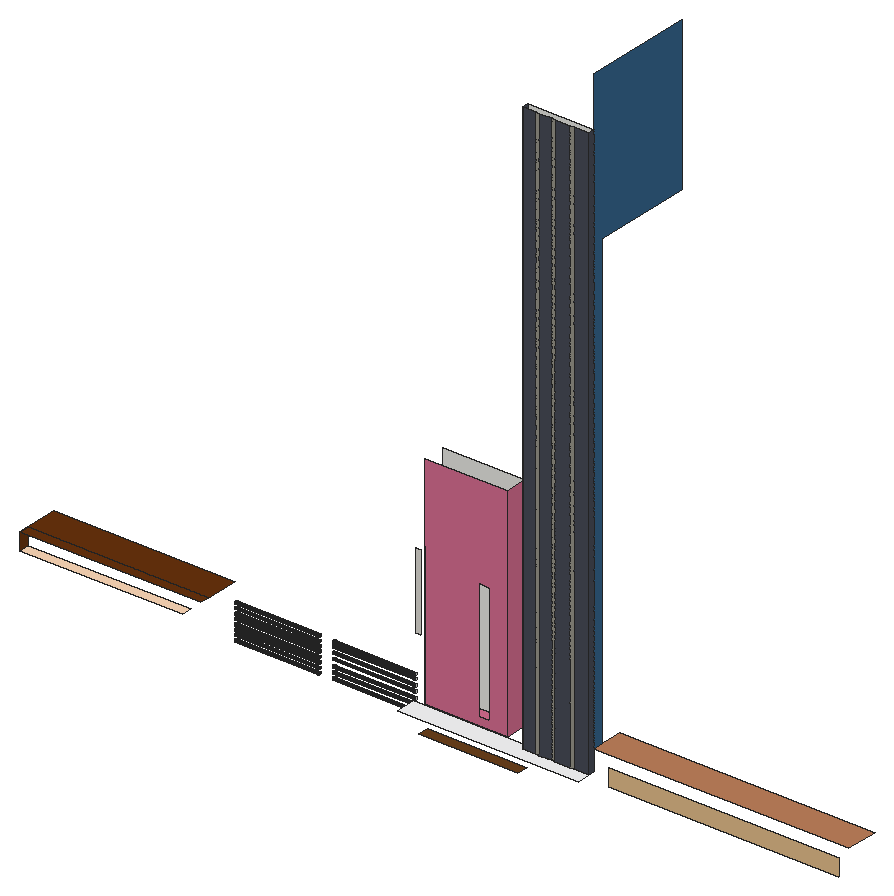
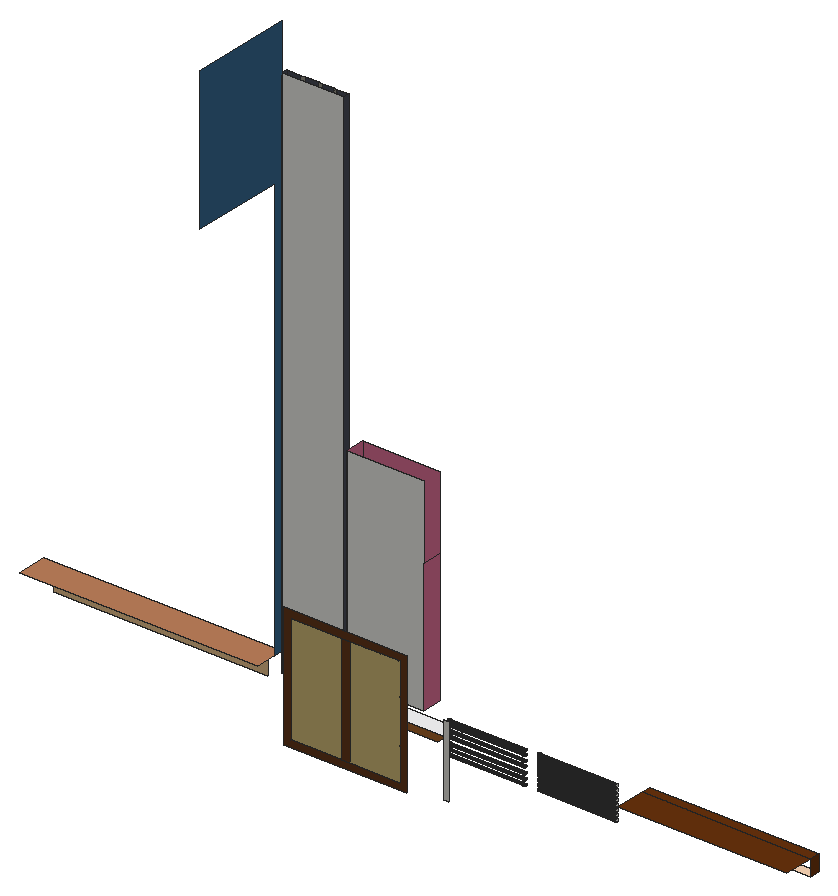
# SketchUp Ruby script. Lengths in inches.
U = 1.inch
M = Sketchup.active_model
def pt(a) = Geom::Point3d.new(a.map { |v| v * U })
def face(e, loops, mat)
  f = e.add_face(loops[0].map { |a| pt(a) })
  loops[1..].each { |l| e.add_face(l.map { |a| pt(a) }).erase! }
  f.material = f.back_material = mat if mat
  f
end
# faces: each face lists its corners as indices into pts; further lists are holes
def faces(e, pts, list, mat = nil) = list.each { |f| face(e, (f[0].is_a?(Array) ? f : [f]).map { |l| l.map { |i| pts[i] } }, mat) }
# xy, xz, yz: faces in a plane at the given z, y or x. An outline is a flat list of corners, or four numbers for a rectangle; further outlines are holes
def ring(l) = l.size == 4 ? [[l[0], l[1]], [l[2], l[1]], [l[2], l[3]], [l[0], l[3]]] : l.each_slice(2).to_a
def flat(e, list, mat, &to3) = list.each { |f| face(e, (f[0].is_a?(Array) ? f : [f]).map { |l| ring(l).map { |u, v| to3.(u, v) } }, mat) }
def xy(e, z, list, mat = nil) = flat(e, list, mat) { |x, y| [x, y, z] }
def xz(e, y, list, mat = nil) = flat(e, list, mat) { |x, z| [x, y, z] }
def yz(e, x, list, mat = nil) = flat(e, list, mat) { |y, z| [x, y, z] }
def lines(e, pts, list) = list.each { |a, b| e.add_line(pt(pts[a]), pt(pts[b])) }
# prism: a flat outline (further loops are holes) pulled along v
def prism(e, loops, v, mat = nil)
  f = face(e, loops, mat); d = Geom::Vector3d.new(v.map { |x| x * U })
  f.pushpull(f.normal.samedirection?(d) ? d.length : -d.length)
end
def box(e, o, s, mat = nil) = prism(e, [[o, [o[0] + s[0], o[1], o[2]], [o[0] + s[0], o[1] + s[1], o[2]], [o[0], o[1] + s[1], o[2]]]], [0, 0, s[2]], mat)
def at(x, y, z, deg = 0) = Geom::Transformation.translation(pt([x, y, z])) * Geom::Transformation.rotation(ORIGIN, Z_AXIS, deg.degrees)
def axes(o, x, y, z) = Geom::Transformation.new([*x, 0, *y, 0, *z, 0, *pt(o).to_a, 1])
def part(name) = M.definitions.add(name)
# library, detail: a bought-in or finely detailed component or shape, given as its bounding box
def library(name, o, s) = part(name).tap { |d| box(d.entities, o, s) }
def detail(e, o, s) = box(e.add_group.entities, o, s)
def put(e, d, t, mat = nil) = e.add_instance(d, t).tap { |i| i.material = mat if mat }
def group(e, t, mat = nil) = e.add_group.tap { |g| g.transformation = t; g.material = mat if mat }.entities
root = M.entities
M.materials.add("[0001_PaleVioletRed]").color = [211, 108, 142]
M.materials.add("[0027_PeachPuff]").color = [255, 218, 185]
M.materials.add("[0036_BurlyWood]").color = [222, 184, 135]
M.materials.add("[0043_SaddleBrown]").color = [104, 51, 14]
M.materials.add("[0100_SteelBlue]").color = [53, 99, 137]
M.materials.add("[Formica Graystone]").color = [149, 146, 135]
M.materials.add("[Formica Laminate Dark]").color = [70, 74, 84]
M.materials.add("[Polished Concrete New]").color = [200, 200, 203]
M.materials.add("[Quartz Light Grey]").color = [251, 251, 252]
M.materials.add("[Terrazzo Tile Light]").color = [219, 217, 210]
M.materials.add("[Window Covering 02]").color = [199, 178, 115]
M.materials.add("[Wood Cherry Original]").color = [96, 54, 26]
M.materials.add("[Wood Floor Parquet]").color = [107, 65, 28]
M.materials.add("[Wood Veneer 02]").color = [190, 128, 91]
xy(root,37.8125,[[216.35,107.04,269.29,112.73]],"[Wood Floor Parquet]")
xy(root,44.875,[[266.37,114.04,301.48,117.35]])
xy(root,44.875,[[205.34,107.04,301.48,107.04,301.48,114.04,266.37,114.04,266.37,117.35,205.34,117.35]],"[Quartz Light Grey]")
xy(root,47.01,[[0,112.04,86.375,117.35]],"[0027_PeachPuff]")
xy(root,53.88,[[220.625,105.92,264.66,117.35]],"[0001_PaleVioletRed]")
xy(root,56.125,[[0,112.04,96.16,117.35],[0,117.35,96.16,134.6]],"[0043_SaddleBrown]")
xy(root,56.125,[[301.48,117.35,437.01,134.6]],"[Wood Veneer 02]")
xz(root,105.92,[[[220.625,53.88,264.66,171.19],[248.98,57.97,254.98,121.72]]],"[0001_PaleVioletRed]")
xz(root,114.04,[[272.89,44.875,274.86,351.35],[281.39,44.875,283.36,351.35],[291.26,44.875,293.24,351.35]],"[Formica Graystone]")
xz(root,114.04,[[266.37,44.875,272.89,351.35],[274.86,44.875,281.39,351.35],[283.36,44.875,291.26,351.35],[293.24,44.875,301.48,351.35]],"[Formica Laminate Dark]")
xz(root,117.35,[[266.37,44.875,301.48,351.35],[220.625,53.88,264.66,171.19]])
xz(root,117.35,[[309.46,40.81,431.59,49.875]],"[0036_BurlyWood]")
xz(root,162.72,[[170.43,45.29,173.12,85.79]],"[Terrazzo Tile Light]")
xz(root,162.72,[[198.18,45.28,226.54,107.29],[230.91,45.28,260.19,107.29]],"[Window Covering 02]")
xz(root,162.72,[[[194.0625,41.16,264.3125,111.41],[198.18,45.28,260.19,107.29]],[226.54,45.28,230.91,107.29]],"[Wood Cherry Original]")
yz(root,0,[[112.04,47.01,117.35,56.125]],"[0043_SaddleBrown]")
yz(root,108.27,[[120.22,38.1,120.06,38.12,119.91,38.18,119.78,38.28,119.68,38.41,119.61,38.5625,119.59,38.72,119.61,38.88,119.68,39.04,119.78,39.16,119.91,39.26,120.06,39.33,120.22,39.35,120.38,39.33,120.53,39.26,120.66,39.16,120.76,39.04,120.82,38.88,120.84,38.72,120.82,38.5625,120.76,38.41,120.66,38.28,120.53,38.18,120.38,38.12],[120.22,40.66,120.06,40.68,119.91,40.74,119.78,40.84,119.68,40.97,119.61,41.125,119.59,41.29,119.61,41.45,119.68,41.6,119.78,41.73,119.91,41.83,120.06,41.89,120.22,41.91,120.38,41.89,120.53,41.83,120.66,41.73,120.76,41.6,120.82,41.45,120.84,41.29,120.82,41.125,120.76,40.97,120.66,40.84,120.53,40.74,120.38,40.68],[120.22,43.22,120.06,43.24,119.91,43.31,119.78,43.41,119.68,43.54,119.61,43.6875,119.59,43.85,119.61,44.01,119.68,44.16,119.78,44.29,119.91,44.39,120.06,44.45,120.22,44.47,120.38,44.45,120.53,44.39,120.66,44.29,120.76,44.16,120.82,44.01,120.84,43.85,120.82,43.6875,120.76,43.54,120.66,43.41,120.53,43.31,120.38,43.24],[120.22,45.79,120.06,45.81,119.91,45.87,119.78,45.97,119.68,46.1,119.61,46.25,119.59,46.41,119.61,46.57,119.68,46.72,119.78,46.85,119.91,46.95,120.06,47.01,120.22,47.04,120.38,47.01,120.53,46.95,120.66,46.85,120.76,46.72,120.82,46.57,120.84,46.41,120.82,46.25,120.76,46.1,120.66,45.97,120.53,45.87,120.38,45.81],[120.22,48.35,120.06,48.37,119.91,48.43,119.78,48.53,119.68,48.66,119.61,48.8125,119.59,48.97,119.61,49.13,119.68,49.29,119.78,49.41,119.91,49.51,120.06,49.58,120.22,49.6,120.38,49.58,120.53,49.51,120.66,49.41,120.76,49.29,120.82,49.13,120.84,48.97,120.82,48.8125,120.76,48.66,120.66,48.53,120.53,48.43,120.38,48.37],
  [120.22,50.91,120.06,50.93,119.91,50.99,119.78,51.09,119.68,51.22,119.61,51.375,119.59,51.54,119.61,51.7,119.68,51.85,119.78,51.98,119.91,52.08,120.06,52.14,120.22,52.16,120.38,52.14,120.53,52.08,120.66,51.98,120.76,51.85,120.82,51.7,120.84,51.54,120.82,51.375,120.76,51.22,120.66,51.09,120.53,50.99,120.38,50.93],[120.22,53.47,120.06,53.49,119.91,53.56,119.78,53.66,119.68,53.79,119.61,53.9375,119.59,54.1,119.61,54.26,119.68,54.41,119.78,54.54,119.91,54.64,120.06,54.7,120.22,54.72,120.38,54.7,120.53,54.64,120.66,54.54,120.76,54.41,120.82,54.26,120.84,54.1,120.82,53.9375,120.76,53.79,120.66,53.66,120.53,53.56,120.38,53.49],[120.22,56.04,120.06,56.06,119.91,56.12,119.78,56.22,119.68,56.35,119.61,56.5,119.59,56.66,119.61,56.82,119.68,56.97,119.78,57.1,119.91,57.2,120.06,57.26,120.22,57.29,120.38,57.26,120.53,57.2,120.66,57.1,120.76,56.97,120.82,56.82,120.84,56.66,120.82,56.5,120.76,56.35,120.66,56.22,120.53,56.12,120.38,56.06]])
yz(root,204.4,[[120.29,38.04,120.45,38.0625,120.6,38.125,120.73,38.22,120.83,38.35,120.89,38.5,120.91,38.66,120.89,38.83,120.83,38.98,120.73,39.11,120.6,39.21,120.45,39.27,120.29,39.29,120.13,39.27,119.98,39.21,119.85,39.11,119.75,38.98,119.6875,38.83,119.66,38.66,119.6875,38.5,119.75,38.35,119.85,38.22,119.98,38.125,120.13,38.0625],[120.29,41.04,120.45,41.0625,120.6,41.125,120.73,41.22,120.83,41.35,120.89,41.5,120.91,41.66,120.89,41.83,120.83,41.98,120.73,42.11,120.6,42.21,120.45,42.27,120.29,42.29,120.13,42.27,119.98,42.21,119.85,42.11,119.75,41.98,119.6875,41.83,119.66,41.66,119.6875,41.5,119.75,41.35,119.85,41.22,119.98,41.125,120.13,41.0625],[120.29,43.91,120.45,43.9375,120.6,44,120.73,44.1,120.83,44.23,120.89,44.38,120.91,44.54,120.89,44.7,120.83,44.85,120.73,44.98,120.6,45.08,120.45,45.14,120.29,45.16,120.13,45.14,119.98,45.08,119.85,44.98,119.75,44.85,119.6875,44.7,119.66,44.54,119.6875,44.38,119.75,44.23,119.85,44.1,119.98,44,120.13,43.9375],[120.29,47.41,120.45,47.4375,120.6,47.5,120.73,47.6,120.83,47.73,120.89,47.88,120.91,48.04,120.89,48.2,120.83,48.35,120.73,48.48,120.6,48.58,120.45,48.64,120.29,48.66,120.13,48.64,119.98,48.58,119.85,48.48,119.75,48.35,119.6875,48.2,119.66,48.04,119.6875,47.88,119.75,47.73,119.85,47.6,119.98,47.5,120.13,47.4375],[120.29,50.29,120.45,50.3125,120.6,50.375,120.73,50.47,120.83,50.6,120.89,50.75,120.91,50.91,120.89,51.08,120.83,51.23,120.73,51.36,120.6,51.46,120.45,51.52,120.29,51.54,120.13,51.52,119.98,51.46,119.85,51.36,119.75,51.23,119.6875,51.08,119.66,50.91,119.6875,50.75,119.75,50.6,119.85,50.47,119.98,50.375,120.13,50.3125],
  [120.29,53.35,120.45,53.375,120.6,53.4375,120.73,53.54,120.83,53.66,120.89,53.82,120.91,53.98,120.89,54.14,120.83,54.29,120.73,54.42,120.6,54.52,120.45,54.58,120.29,54.6,120.13,54.58,119.98,54.52,119.85,54.42,119.75,54.29,119.6875,54.14,119.66,53.98,119.6875,53.82,119.75,53.66,119.85,53.54,119.98,53.4375,120.13,53.375],[120.29,55.6,120.45,55.625,120.6,55.6875,120.73,55.79,120.83,55.91,120.89,56.07,120.91,56.23,120.89,56.39,120.83,56.54,120.73,56.67,120.6,56.77,120.45,56.83,120.29,56.85,120.13,56.83,119.98,56.77,119.85,56.67,119.75,56.54,119.6875,56.39,119.66,56.23,119.6875,56.07,119.75,55.91,119.85,55.79,119.98,55.6875,120.13,55.625]])
yz(root,220.625,[[105.92,53.88,117.35,129]],"[0001_PaleVioletRed]")
yz(root,264.66,[[105.92,53.88,117.35,171.19]],"[0001_PaleVioletRed]")
yz(root,266.37,[[114.04,44.875,117.35,351.35]],"[Formica Laminate Dark]")
yz(root,301.48,[[117.35,56.125,122.78,56.125,122.78,297,175.59,297,175.59,378.0625,117.35,378.0625]],"[0100_SteelBlue]")
yz(root,301.48,[[114.04,44.875,117.35,351.35]],"[Formica Laminate Dark]")
p = [[204.4,120.29,38.04],[204.4,120.13,38.0625],[160.24,120.13,38.0625],[160.24,120.29,38.04],[204.4,120.45,38.0625],[160.24,120.45,38.0625],
  [204.4,119.98,38.125],[204.4,119.85,38.22],[160.24,119.85,38.22],[160.24,119.98,38.125],[108.27,119.91,38.18],[108.27,120.06,38.12],
  [153.22,120.06,38.12],[153.22,119.91,38.18],[108.27,120.22,38.1],[153.22,120.22,38.1],[108.27,120.38,38.12],[153.22,120.38,38.12],
  [108.27,120.53,38.18],[153.22,120.53,38.18],[204.4,120.6,38.125],[160.24,120.6,38.125],[204.4,120.73,38.22],[160.24,120.73,38.22],
  [204.4,119.75,38.35],[160.24,119.75,38.35],[108.27,119.78,38.28],[153.22,119.78,38.28],[108.27,120.66,38.28],[153.22,120.66,38.28],
  [204.4,120.83,38.35],[160.24,120.83,38.35],[108.27,119.68,38.41],[153.22,119.68,38.41],[108.27,120.76,38.41],[153.22,120.76,38.41],
  [108.27,119.61,38.5625],[153.22,119.61,38.5625],[204.4,119.6875,38.5],[160.24,119.6875,38.5],[108.27,120.82,38.5625],[153.22,120.82,38.5625],
  [204.4,120.89,38.5],[160.24,120.89,38.5],[204.4,119.66,38.66],[160.24,119.66,38.66],[204.4,120.91,38.66],[160.24,120.91,38.66],
  [108.27,119.59,38.72],[153.22,119.59,38.72],[108.27,120.84,38.72],[153.22,120.84,38.72],[108.27,119.61,38.88],[153.22,119.61,38.88],
  [204.4,119.6875,38.83],[160.24,119.6875,38.83],[108.27,120.82,38.88],[153.22,120.82,38.88],[204.4,120.89,38.83],[160.24,120.89,38.83],
  [204.4,119.75,38.98],[160.24,119.75,38.98],[204.4,120.83,38.98],[160.24,120.83,38.98],[108.27,119.68,39.04],[153.22,119.68,39.04],
  [108.27,120.76,39.04],[153.22,120.76,39.04],[108.27,119.78,39.16],[153.22,119.78,39.16],[204.4,119.85,39.11],[160.24,119.85,39.11],
  [108.27,120.66,39.16],[153.22,120.66,39.16],[204.4,120.73,39.11],[160.24,120.73,39.11],[204.4,119.98,39.21],[160.24,119.98,39.21],
  [204.4,120.6,39.21],[160.24,120.6,39.21],[108.27,119.91,39.26],[153.22,119.91,39.26],[204.4,120.13,39.27],[160.24,120.13,39.27],
  [108.27,120.53,39.26],[153.22,120.53,39.26],[204.4,120.45,39.27],[160.24,120.45,39.27],[108.27,120.06,39.33],[153.22,120.06,39.33],
  [108.27,120.22,39.35],[153.22,120.22,39.35],[204.4,120.29,39.29],[160.24,120.29,39.29],[108.27,120.38,39.33],[153.22,120.38,39.33],
  [108.27,119.78,40.84],[108.27,119.91,40.74],[153.22,119.91,40.74],[153.22,119.78,40.84],[108.27,120.06,40.68],[153.22,120.06,40.68],
  [108.27,120.22,40.66],[153.22,120.22,40.66],[108.27,120.38,40.68],[153.22,120.38,40.68],[108.27,120.53,40.74],[153.22,120.53,40.74],
  [108.27,120.66,40.84],[153.22,120.66,40.84],[108.27,119.68,40.97],[153.22,119.68,40.97],[108.27,120.76,40.97],[153.22,120.76,40.97],
  [108.27,119.61,41.125],[153.22,119.61,41.125],[204.4,120.29,41.04],[204.4,120.13,41.0625],[160.24,120.13,41.0625],[160.24,120.29,41.04],
  [204.4,120.45,41.0625],[160.24,120.45,41.0625],[108.27,120.82,41.125],[153.22,120.82,41.125],[108.27,119.59,41.29],[153.22,119.59,41.29],
  [204.4,119.98,41.125],[204.4,119.85,41.22],[160.24,119.85,41.22],[160.24,119.98,41.125],[204.4,120.6,41.125],[160.24,120.6,41.125],
  [204.4,120.73,41.22],[160.24,120.73,41.22],[108.27,120.84,41.29],[153.22,120.84,41.29],[204.4,119.75,41.35],[160.24,119.75,41.35],
  [204.4,120.83,41.35],[160.24,120.83,41.35],[108.27,119.61,41.45],[153.22,119.61,41.45],[108.27,120.82,41.45],[153.22,120.82,41.45],
  [108.27,119.68,41.6],[153.22,119.68,41.6],[204.4,119.6875,41.5],[160.24,119.6875,41.5],[108.27,120.76,41.6],[153.22,120.76,41.6],
  [204.4,120.89,41.5],[160.24,120.89,41.5],[204.4,119.66,41.66],[160.24,119.66,41.66],[204.4,120.91,41.66],[160.24,120.91,41.66],
  [108.27,119.78,41.73],[153.22,119.78,41.73],[108.27,120.66,41.73],[153.22,120.66,41.73],[204.4,119.6875,41.83],[160.24,119.6875,41.83],
  [108.27,119.91,41.83],[153.22,119.91,41.83],[108.27,120.53,41.83],[153.22,120.53,41.83],[204.4,120.89,41.83],[160.24,120.89,41.83],
  [204.4,119.75,41.98],[160.24,119.75,41.98],[108.27,120.06,41.89],[153.22,120.06,41.89],[108.27,120.38,41.89],[153.22,120.38,41.89],
  [204.4,120.83,41.98],[160.24,120.83,41.98],[108.27,120.22,41.91],[153.22,120.22,41.91],[204.4,119.85,42.11],[160.24,119.85,42.11],
  [204.4,120.73,42.11],[160.24,120.73,42.11],[204.4,119.98,42.21],[160.24,119.98,42.21],[204.4,120.6,42.21],[160.24,120.6,42.21],
  [204.4,120.13,42.27],[160.24,120.13,42.27],[204.4,120.45,42.27],[160.24,120.45,42.27],[204.4,120.29,42.29],[160.24,120.29,42.29],
  [108.27,119.91,43.31],[108.27,120.06,43.24],[153.22,120.06,43.24],[153.22,119.91,43.31],[108.27,120.22,43.22],[153.22,120.22,43.22],
  [108.27,120.38,43.24],[153.22,120.38,43.24],[108.27,120.53,43.31],[153.22,120.53,43.31],[108.27,119.78,43.41],[153.22,119.78,43.41],
  [108.27,120.66,43.41],[153.22,120.66,43.41],[108.27,119.68,43.54],[153.22,119.68,43.54],[108.27,120.76,43.54],[153.22,120.76,43.54],
  [108.27,119.61,43.6875],[153.22,119.61,43.6875],[108.27,120.82,43.6875],[153.22,120.82,43.6875],[108.27,119.59,43.85],[153.22,119.59,43.85],
  [108.27,120.84,43.85],[153.22,120.84,43.85],[108.27,119.61,44.01],[153.22,119.61,44.01],[108.27,120.82,44.01],[153.22,120.82,44.01],
  [204.4,120.13,43.9375],[204.4,119.98,44],[160.24,119.98,44],[160.24,120.13,43.9375],[204.4,120.29,43.91],[160.24,120.29,43.91],
  [204.4,120.45,43.9375],[160.24,120.45,43.9375],[204.4,120.6,44],[160.24,120.6,44],[108.27,119.68,44.16],[153.22,119.68,44.16],
  [204.4,119.85,44.1],[160.24,119.85,44.1],[204.4,120.73,44.1],[160.24,120.73,44.1],[108.27,120.76,44.16],[153.22,120.76,44.16],
  [204.4,119.75,44.23],[160.24,119.75,44.23],[204.4,120.83,44.23],[160.24,120.83,44.23],[108.27,119.78,44.29],[153.22,119.78,44.29],
  [204.4,119.6875,44.38],[160.24,119.6875,44.38],[108.27,120.66,44.29],[153.22,120.66,44.29],[204.4,120.89,44.38],[160.24,120.89,44.38],
  [108.27,119.91,44.39],[153.22,119.91,44.39],[108.27,120.53,44.39],[153.22,120.53,44.39],[204.4,119.66,44.54],[160.24,119.66,44.54],
  [108.27,120.06,44.45],[153.22,120.06,44.45],[108.27,120.38,44.45],[153.22,120.38,44.45],[204.4,120.91,44.54],[160.24,120.91,44.54],
  [204.4,119.6875,44.7],[160.24,119.6875,44.7],[108.27,120.22,44.47],[153.22,120.22,44.47],[204.4,120.89,44.7],[160.24,120.89,44.7],
  [204.4,119.75,44.85],[160.24,119.75,44.85],[204.4,120.83,44.85],[160.24,120.83,44.85],[204.4,119.85,44.98],[160.24,119.85,44.98],
  [204.4,120.73,44.98],[160.24,120.73,44.98],[204.4,119.98,45.08],[160.24,119.98,45.08],[204.4,120.6,45.08],[160.24,120.6,45.08],
  [204.4,120.13,45.14],[160.24,120.13,45.14],[204.4,120.29,45.16],[160.24,120.29,45.16],[204.4,120.45,45.14],[160.24,120.45,45.14],
  [108.27,119.91,45.87],[108.27,120.06,45.81],[153.22,120.06,45.81],[153.22,119.91,45.87],[108.27,120.22,45.79],[153.22,120.22,45.79],
  [108.27,120.38,45.81],[153.22,120.38,45.81],[108.27,120.53,45.87],[153.22,120.53,45.87],[108.27,119.78,45.97],[153.22,119.78,45.97],
  [108.27,120.66,45.97],[153.22,120.66,45.97],[108.27,119.68,46.1],[153.22,119.68,46.1],[108.27,120.76,46.1],[153.22,120.76,46.1],
  [108.27,119.61,46.25],[153.22,119.61,46.25],[108.27,120.82,46.25],[153.22,120.82,46.25],[108.27,119.59,46.41],[153.22,119.59,46.41],
  [108.27,120.84,46.41],[153.22,120.84,46.41],[108.27,119.61,46.57],[153.22,119.61,46.57],[108.27,120.82,46.57],[153.22,120.82,46.57],
  [108.27,119.68,46.72],[153.22,119.68,46.72],[108.27,120.76,46.72],[153.22,120.76,46.72],[108.27,119.78,46.85],[153.22,119.78,46.85],
  [108.27,120.66,46.85],[153.22,120.66,46.85],[108.27,119.91,46.95],[153.22,119.91,46.95],[108.27,120.53,46.95],[153.22,120.53,46.95],
  [108.27,120.06,47.01],[153.22,120.06,47.01],[108.27,120.22,47.04],[153.22,120.22,47.04],[108.27,120.38,47.01],[153.22,120.38,47.01],
  [204.4,120.13,47.4375],[204.4,119.98,47.5],[160.24,119.98,47.5],[160.24,120.13,47.4375],[204.4,120.29,47.41],[160.24,120.29,47.41],
  [204.4,120.45,47.4375],[160.24,120.45,47.4375],[204.4,120.6,47.5],[160.24,120.6,47.5],[204.4,119.85,47.6],[160.24,119.85,47.6],
  [204.4,120.73,47.6],[160.24,120.73,47.6],[204.4,119.75,47.73],[160.24,119.75,47.73],[204.4,120.83,47.73],[160.24,120.83,47.73],
  [204.4,119.6875,47.88],[160.24,119.6875,47.88],[204.4,120.89,47.88],[160.24,120.89,47.88],[204.4,119.66,48.04],[160.24,119.66,48.04],
  [204.4,120.91,48.04],[160.24,120.91,48.04],[204.4,119.6875,48.2],[160.24,119.6875,48.2],[204.4,120.89,48.2],[160.24,120.89,48.2],
  [204.4,119.75,48.35],[160.24,119.75,48.35],[204.4,120.83,48.35],[160.24,120.83,48.35],[108.27,120.06,48.37],[108.27,120.22,48.35],
  [153.22,120.22,48.35],[153.22,120.06,48.37],[108.27,120.38,48.37],[153.22,120.38,48.37],[204.4,119.85,48.48],[160.24,119.85,48.48],
  [108.27,119.78,48.53],[108.27,119.91,48.43],[153.22,119.91,48.43],[153.22,119.78,48.53],[108.27,120.53,48.43],[153.22,120.53,48.43],
  [108.27,120.66,48.53],[153.22,120.66,48.53],[204.4,120.73,48.48],[160.24,120.73,48.48],[108.27,119.68,48.66],[153.22,119.68,48.66],
  [204.4,119.98,48.58],[160.24,119.98,48.58],[204.4,120.6,48.58],[160.24,120.6,48.58],[108.27,120.76,48.66],[153.22,120.76,48.66],
  [204.4,120.13,48.64],[160.24,120.13,48.64],[204.4,120.29,48.66],[160.24,120.29,48.66],[204.4,120.45,48.64],[160.24,120.45,48.64],
  [108.27,119.61,48.8125],[153.22,119.61,48.8125],[108.27,120.82,48.8125],[153.22,120.82,48.8125],[108.27,119.59,48.97],[153.22,119.59,48.97],
  [108.27,120.84,48.97],[153.22,120.84,48.97],[108.27,119.61,49.13],[153.22,119.61,49.13],[108.27,120.82,49.13],[153.22,120.82,49.13],
  [108.27,119.68,49.29],[153.22,119.68,49.29],[108.27,120.76,49.29],[153.22,120.76,49.29],[108.27,119.78,49.41],[153.22,119.78,49.41],
  [108.27,120.66,49.41],[153.22,120.66,49.41],[108.27,119.91,49.51],[153.22,119.91,49.51],[108.27,120.53,49.51],[153.22,120.53,49.51],
  [108.27,120.06,49.58],[153.22,120.06,49.58],[108.27,120.38,49.58],[153.22,120.38,49.58],[108.27,120.22,49.6],[153.22,120.22,49.6],
  [204.4,120.13,50.3125],[204.4,119.98,50.375],[160.24,119.98,50.375],[160.24,120.13,50.3125],[204.4,120.29,50.29],[160.24,120.29,50.29],
  [204.4,120.45,50.3125],[160.24,120.45,50.3125],[204.4,120.6,50.375],[160.24,120.6,50.375],[204.4,119.85,50.47],[160.24,119.85,50.47],
  [204.4,120.73,50.47],[160.24,120.73,50.47],[204.4,119.75,50.6],[160.24,119.75,50.6],[204.4,120.83,50.6],[160.24,120.83,50.6],
  [204.4,119.6875,50.75],[160.24,119.6875,50.75],[204.4,120.89,50.75],[160.24,120.89,50.75],[204.4,119.66,50.91],[160.24,119.66,50.91],
  [204.4,120.91,50.91],[160.24,120.91,50.91],[204.4,119.6875,51.08],[160.24,119.6875,51.08],[108.27,119.91,50.99],[108.27,120.06,50.93],
  [153.22,120.06,50.93],[153.22,119.91,50.99],[108.27,120.22,50.91],[153.22,120.22,50.91],[108.27,120.38,50.93],[153.22,120.38,50.93],
  [108.27,120.53,50.99],[153.22,120.53,50.99],[204.4,120.89,51.08],[160.24,120.89,51.08],[108.27,119.78,51.09],[153.22,119.78,51.09],
  [108.27,120.66,51.09],[153.22,120.66,51.09],[108.27,119.68,51.22],[153.22,119.68,51.22],[204.4,119.75,51.23],[160.24,119.75,51.23],
  [108.27,120.76,51.22],[153.22,120.76,51.22],[204.4,120.83,51.23],[160.24,120.83,51.23],[108.27,119.61,51.375],[153.22,119.61,51.375],
  [204.4,119.85,51.36],[160.24,119.85,51.36],[204.4,120.73,51.36],[160.24,120.73,51.36],[108.27,120.82,51.375],[153.22,120.82,51.375],
  [108.27,119.59,51.54],[153.22,119.59,51.54],[204.4,119.98,51.46],[160.24,119.98,51.46],[204.4,120.6,51.46],[160.24,120.6,51.46],
  [108.27,120.84,51.54],[153.22,120.84,51.54],[108.27,119.61,51.7],[153.22,119.61,51.7],[204.4,120.13,51.52],[160.24,120.13,51.52],
  [204.4,120.29,51.54],[160.24,120.29,51.54],[204.4,120.45,51.52],[160.24,120.45,51.52],[108.27,120.82,51.7],[153.22,120.82,51.7],
  [108.27,119.68,51.85],[153.22,119.68,51.85],[108.27,120.76,51.85],[153.22,120.76,51.85],[108.27,119.78,51.98],[153.22,119.78,51.98],
  [108.27,120.66,51.98],[153.22,120.66,51.98],[108.27,119.91,52.08],[153.22,119.91,52.08],[108.27,120.53,52.08],[153.22,120.53,52.08],
  [108.27,120.06,52.14],[153.22,120.06,52.14],[108.27,120.22,52.16],[153.22,120.22,52.16],[108.27,120.38,52.14],[153.22,120.38,52.14],
  [204.4,119.98,53.4375],[204.4,119.85,53.54],[160.24,119.85,53.54],[160.24,119.98,53.4375],[204.4,120.13,53.375],[160.24,120.13,53.375],
  [204.4,120.29,53.35],[160.24,120.29,53.35],[204.4,120.45,53.375],[160.24,120.45,53.375],[204.4,120.6,53.4375],[160.24,120.6,53.4375],
  [204.4,120.73,53.54],[160.24,120.73,53.54],[204.4,119.75,53.66],[160.24,119.75,53.66],[108.27,119.91,53.56],[108.27,120.06,53.49],
  [153.22,120.06,53.49],[153.22,119.91,53.56],[108.27,120.22,53.47],[153.22,120.22,53.47],[108.27,120.38,53.49],[153.22,120.38,53.49],
  [108.27,120.53,53.56],[153.22,120.53,53.56],[204.4,120.83,53.66],[160.24,120.83,53.66],[108.27,119.78,53.66],[153.22,119.78,53.66],
  [108.27,120.66,53.66],[153.22,120.66,53.66],[108.27,119.68,53.79],[153.22,119.68,53.79],[204.4,119.6875,53.82],[160.24,119.6875,53.82],
  [108.27,120.76,53.79],[153.22,120.76,53.79],[204.4,120.89,53.82],[160.24,120.89,53.82],[108.27,119.61,53.9375],[153.22,119.61,53.9375],
  [204.4,119.66,53.98],[160.24,119.66,53.98],[108.27,120.82,53.9375],[153.22,120.82,53.9375],[204.4,120.91,53.98],[160.24,120.91,53.98],
  [108.27,119.59,54.1],[153.22,119.59,54.1],[108.27,120.84,54.1],[153.22,120.84,54.1],[204.4,119.6875,54.14],[160.24,119.6875,54.14],
  [204.4,120.89,54.14],[160.24,120.89,54.14],[108.27,119.61,54.26],[153.22,119.61,54.26],[204.4,119.75,54.29],[160.24,119.75,54.29],
  [108.27,120.82,54.26],[153.22,120.82,54.26],[204.4,120.83,54.29],[160.24,120.83,54.29],[108.27,119.68,54.41],[153.22,119.68,54.41],
  [204.4,119.85,54.42],[160.24,119.85,54.42],[204.4,120.73,54.42],[160.24,120.73,54.42],[108.27,120.76,54.41],[153.22,120.76,54.41],
  [108.27,119.78,54.54],[153.22,119.78,54.54],[204.4,119.98,54.52],[160.24,119.98,54.52],[204.4,120.6,54.52],[160.24,120.6,54.52],
  [108.27,120.66,54.54],[153.22,120.66,54.54],[108.27,119.91,54.64],[153.22,119.91,54.64],[204.4,120.13,54.58],[160.24,120.13,54.58],
  [108.27,120.53,54.64],[153.22,120.53,54.64],[204.4,120.45,54.58],[160.24,120.45,54.58],[108.27,120.06,54.7],[153.22,120.06,54.7],
  [204.4,120.29,54.6],[160.24,120.29,54.6],[108.27,120.38,54.7],[153.22,120.38,54.7],[108.27,120.22,54.72],[153.22,120.22,54.72],
  [204.4,120.13,55.625],[204.4,119.98,55.6875],[160.24,119.98,55.6875],[160.24,120.13,55.625],[204.4,120.29,55.6],[160.24,120.29,55.6],
  [204.4,120.45,55.625],[160.24,120.45,55.625],[204.4,120.6,55.6875],[160.24,120.6,55.6875],[204.4,119.85,55.79],[160.24,119.85,55.79],
  [204.4,120.73,55.79],[160.24,120.73,55.79],[204.4,119.75,55.91],[160.24,119.75,55.91],[204.4,120.83,55.91],[160.24,120.83,55.91],
  [204.4,119.6875,56.07],[160.24,119.6875,56.07],[204.4,120.89,56.07],[160.24,120.89,56.07],[108.27,120.06,56.06],[108.27,120.22,56.04],
  [153.22,120.22,56.04],[153.22,120.06,56.06],[108.27,120.38,56.06],[153.22,120.38,56.06],[204.4,119.66,56.23],[160.24,119.66,56.23],
  [108.27,119.78,56.22],[108.27,119.91,56.12],[153.22,119.91,56.12],[153.22,119.78,56.22],[108.27,120.53,56.12],[153.22,120.53,56.12],
  [108.27,120.66,56.22],[153.22,120.66,56.22],[204.4,120.91,56.23],[160.24,120.91,56.23],[108.27,119.68,56.35],[153.22,119.68,56.35],
  [204.4,119.6875,56.39],[160.24,119.6875,56.39],[108.27,120.76,56.35],[153.22,120.76,56.35],[204.4,120.89,56.39],[160.24,120.89,56.39],
  [108.27,119.61,56.5],[153.22,119.61,56.5],[108.27,120.82,56.5],[153.22,120.82,56.5],[204.4,119.75,56.54],[160.24,119.75,56.54],
  [204.4,120.83,56.54],[160.24,120.83,56.54],[108.27,119.59,56.66],[153.22,119.59,56.66],[204.4,119.85,56.67],[160.24,119.85,56.67],
  [204.4,120.73,56.67],[160.24,120.73,56.67],[108.27,120.84,56.66],[153.22,120.84,56.66],[108.27,119.61,56.82],[153.22,119.61,56.82],
  [204.4,119.98,56.77],[160.24,119.98,56.77],[204.4,120.6,56.77],[160.24,120.6,56.77],[108.27,120.82,56.82],[153.22,120.82,56.82],
  [108.27,119.68,56.97],[153.22,119.68,56.97],[204.4,120.13,56.83],[160.24,120.13,56.83],[204.4,120.29,56.85],[160.24,120.29,56.85],
  [204.4,120.45,56.83],[160.24,120.45,56.83],[108.27,120.76,56.97],[153.22,120.76,56.97],[108.27,119.78,57.1],[153.22,119.78,57.1],
  [108.27,120.66,57.1],[153.22,120.66,57.1],[108.27,119.91,57.2],[153.22,119.91,57.2],[108.27,120.53,57.2],[153.22,120.53,57.2],
  [108.27,120.06,57.26],[153.22,120.06,57.26],[108.27,120.38,57.26],[153.22,120.38,57.26],[108.27,120.22,57.29],[153.22,120.22,57.29]]
faces(root,p,[[0,1,2,3],[4,0,3,5],[6,7,8,9],[10,11,12,13],[1,6,9,2],[11,14,15,12],[14,16,17,15],[16,18,19,17],
  [20,4,5,21],[22,20,21,23],[7,24,25,8],[26,10,13,27],[18,28,29,19],[30,22,23,31],[32,26,27,33],[28,34,35,29],
  [36,32,33,37],[24,38,39,25],[34,40,41,35],[42,30,31,43],[38,44,45,39],[46,42,43,47],[48,36,37,49],[40,50,51,41],
  [52,48,49,53],[44,54,55,45],[50,56,57,51],[58,46,47,59],[54,60,61,55],[62,58,59,63],[64,52,53,65],[56,66,67,57],
  [68,64,65,69],[60,70,71,61],[66,72,73,67],[74,62,63,75],[70,76,77,71],[78,74,75,79],[80,68,69,81],[76,82,83,77],
  [72,84,85,73],[86,78,79,87],[88,80,81,89],[90,88,89,91],[82,92,93,83],[94,90,91,95],[92,86,87,93],[84,94,95,85],
  [96,97,98,99],[97,100,101,98],[100,102,103,101],[102,104,105,103],[104,106,107,105],[106,108,109,107],[110,96,99,111],[108,112,113,109],
  [114,110,111,115],[116,117,118,119],[120,116,119,121],[112,122,123,113],[124,114,115,125],[126,127,128,129],[117,126,129,118],[130,120,121,131],
  [132,130,131,133],[122,134,135,123],[127,136,137,128],[138,132,133,139],[140,124,125,141],[134,142,143,135],[144,140,141,145],[136,146,147,137],
  [142,148,149,143],[150,138,139,151],[146,152,153,147],[154,150,151,155],[156,144,145,157],[148,158,159,149],[152,160,161,153],[162,156,157,163],
  [158,164,165,159],[166,154,155,167],[160,168,169,161],[170,162,163,171],[164,172,173,165],[174,166,167,175],[176,170,171,177],[172,176,177,173],
  [168,178,179,169],[180,174,175,181],[178,182,183,179],[184,180,181,185],[182,186,187,183],[188,184,185,189],[186,190,191,187],[190,188,189,191],
  [192,193,194,195],[193,196,197,194],[196,198,199,197],[198,200,201,199],[202,192,195,203],[200,204,205,201],[206,202,203,207],[204,208,209,205],
  [210,206,207,211],[208,212,213,209],[214,210,211,215],[212,216,217,213],[218,214,215,219],[216,220,221,217],[222,223,224,225],[226,222,225,227],
  [228,226,227,229],[230,228,229,231],[232,218,219,233],[223,234,235,224],[236,230,231,237],[220,238,239,221],[234,240,241,235],[242,236,237,243],
  [244,232,233,245],[240,246,247,241],[238,248,249,239],[250,242,243,251],[252,244,245,253],[248,254,255,249],[246,256,257,247],[258,252,253,259],
  [254,260,261,255],[262,250,251,263],[256,264,265,257],[266,258,259,267],[260,266,267,261],[268,262,263,269],[264,270,271,265],[272,268,269,273],
  [270,274,275,271],[276,272,273,277],[274,278,279,275],[280,276,277,281],[278,282,283,279],[282,284,285,283],[284,286,287,285],[286,280,281,287],
  [288,289,290,291],[289,292,293,290],[292,294,295,293],[294,296,297,295],[298,288,291,299],[296,300,301,297],[302,298,299,303],[300,304,305,301],
  [306,302,303,307],[304,308,309,305],[310,306,307,311],[308,312,313,309],[314,310,311,315],[312,316,317,313],[318,314,315,319],[316,320,321,317],
  [322,318,319,323],[320,324,325,321],[326,322,323,327],[324,328,329,325],[330,326,327,331],[332,330,331,333],[334,332,333,335],[328,334,335,329],
  [336,337,338,339],[340,336,339,341],[342,340,341,343],[344,342,343,345],[337,346,347,338],[348,344,345,349],[346,350,351,347],[352,348,349,353],
  [350,354,355,351],[356,352,353,357],[354,358,359,355],[360,356,357,361],[358,362,363,359],[364,360,361,365],[362,366,367,363],[368,364,365,369],
  [370,371,372,373],[371,374,375,372],[366,376,377,367],[378,379,380,381],[379,370,373,380],[374,382,383,375],[382,384,385,383],[386,368,369,387],
  [388,378,381,389],[376,390,391,377],[392,386,387,393],[384,394,395,385],[390,396,397,391],[396,398,399,397],[398,400,401,399],[400,392,393,401],
  [402,388,389,403],[394,404,405,395],[406,402,403,407],[404,408,409,405],[410,406,407,411],[408,412,413,409],[414,410,411,415],[412,416,417,413],
  [418,414,415,419],[416,420,421,417],[422,418,419,423],[420,424,425,421],[426,422,423,427],[424,428,429,425],[430,426,427,431],[428,430,431,429],
  [432,433,434,435],[436,432,435,437],[438,436,437,439],[440,438,439,441],[433,442,443,434],[444,440,441,445],[442,446,447,443],[448,444,445,449],
  [446,450,451,447],[452,448,449,453],[450,454,455,451],[456,452,453,457],[454,458,459,455],[460,461,462,463],[461,464,465,462],[464,466,467,465],
  [466,468,469,467],[470,456,457,471],[472,460,463,473],[468,474,475,469],[476,472,473,477],[458,478,479,459],[474,480,481,475],[482,470,471,483],
  [484,476,477,485],[478,486,487,479],[488,482,483,489],[480,490,491,481],[492,484,485,493],[486,494,495,487],[496,488,489,497],[490,498,499,491],
  [500,492,493,501],[494,502,503,495],[502,504,505,503],[504,506,507,505],[506,496,497,507],[498,508,509,499],[510,500,501,511],[508,512,513,509],
  [514,510,511,515],[512,516,517,513],[518,514,515,519],[516,520,521,517],[522,518,519,523],[524,522,523,525],[526,524,525,527],[520,526,527,521],
  [528,529,530,531],[532,528,531,533],[534,532,533,535],[536,534,535,537],[538,536,537,539],[540,538,539,541],[529,542,543,530],[544,545,546,547],
  [545,548,549,546],[548,550,551,549],[550,552,553,551],[554,540,541,555],[556,544,547,557],[552,558,559,553],[560,556,557,561],[542,562,563,543],
  [558,564,565,559],[566,554,555,567],[568,560,561,569],[562,570,571,563],[564,572,573,565],[574,566,567,575],[576,568,569,577],[572,578,579,573],
  [570,580,581,571],[582,574,575,583],[584,576,577,585],[580,586,587,581],[578,588,589,579],[590,582,583,591],[592,584,585,593],[586,594,595,587],
  [596,590,591,597],[588,598,599,589],[600,592,593,601],[594,602,603,595],[604,596,597,605],[598,606,607,599],[608,600,601,609],[602,610,611,603],
  [606,612,613,607],[614,604,605,615],[616,608,609,617],[610,618,619,611],[618,614,615,619],[612,620,621,613],[622,616,617,623],[620,622,623,621],
  [624,625,626,627],[628,624,627,629],[630,628,629,631],[632,630,631,633],[625,634,635,626],[636,632,633,637],[634,638,639,635],[640,636,637,641],
  [638,642,643,639],[644,640,641,645],[646,647,648,649],[647,650,651,648],[642,652,653,643],[654,655,656,657],[655,646,649,656],[650,658,659,651],
  [658,660,661,659],[662,644,645,663],[664,654,657,665],[652,666,667,653],[660,668,669,661],[670,662,663,671],[672,664,665,673],[668,674,675,669],
  [666,676,677,667],[678,670,671,679],[680,672,673,681],[676,682,683,677],[684,678,679,685],[674,686,687,675],[688,680,681,689],[682,690,691,683],
  [692,684,685,693],[686,694,695,687],[696,688,689,697],[690,698,699,691],[698,700,701,699],[700,702,703,701],[702,692,693,703],[694,704,705,695],
  [706,696,697,707],[704,708,709,705],[710,706,707,711],[708,712,713,709],[714,710,711,715],[712,716,717,713],[718,714,715,719],[716,718,719,717]],"[Polished Concrete New]")
